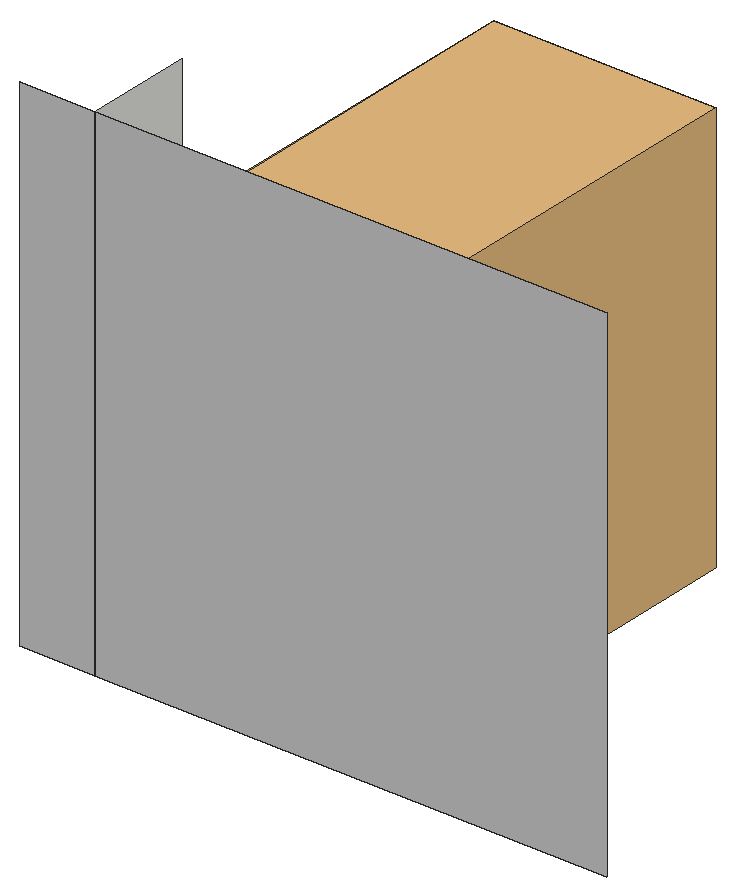
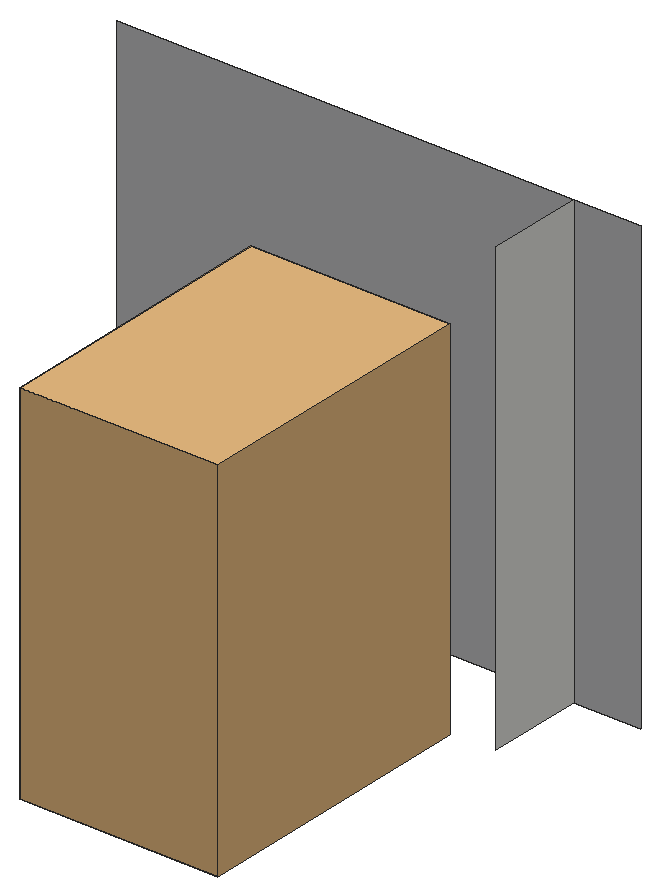
# SketchUp Ruby script. Lengths in inches.
U = 1.inch
M = Sketchup.active_model
def pt(a) = Geom::Point3d.new(a.map { |v| v * U })
def face(e, loops, mat)
  f = e.add_face(loops[0].map { |a| pt(a) })
  loops[1..].each { |l| e.add_face(l.map { |a| pt(a) }).erase! }
  f.material = f.back_material = mat if mat
  f
end
# faces: each face lists its corners as indices into pts; further lists are holes
def faces(e, pts, list, mat = nil) = list.each { |f| face(e, (f[0].is_a?(Array) ? f : [f]).map { |l| l.map { |i| pts[i] } }, mat) }
# xy, xz, yz: faces in a plane at the given z, y or x. An outline is a flat list of corners, or four numbers for a rectangle; further outlines are holes
def ring(l) = l.size == 4 ? [[l[0], l[1]], [l[2], l[1]], [l[2], l[3]], [l[0], l[3]]] : l.each_slice(2).to_a
def flat(e, list, mat, &to3) = list.each { |f| face(e, (f[0].is_a?(Array) ? f : [f]).map { |l| ring(l).map { |u, v| to3.(u, v) } }, mat) }
def xy(e, z, list, mat = nil) = flat(e, list, mat) { |x, y| [x, y, z] }
def xz(e, y, list, mat = nil) = flat(e, list, mat) { |x, z| [x, y, z] }
def yz(e, x, list, mat = nil) = flat(e, list, mat) { |y, z| [x, y, z] }
def lines(e, pts, list) = list.each { |a, b| e.add_line(pt(pts[a]), pt(pts[b])) }
# prism: a flat outline (further loops are holes) pulled along v
def prism(e, loops, v, mat = nil)
  f = face(e, loops, mat); d = Geom::Vector3d.new(v.map { |x| x * U })
  f.pushpull(f.normal.samedirection?(d) ? d.length : -d.length)
end
def box(e, o, s, mat = nil) = prism(e, [[o, [o[0] + s[0], o[1], o[2]], [o[0] + s[0], o[1] + s[1], o[2]], [o[0], o[1] + s[1], o[2]]]], [0, 0, s[2]], mat)
def at(x, y, z, deg = 0) = Geom::Transformation.translation(pt([x, y, z])) * Geom::Transformation.rotation(ORIGIN, Z_AXIS, deg.degrees)
def axes(o, x, y, z) = Geom::Transformation.new([*x, 0, *y, 0, *z, 0, *pt(o).to_a, 1])
def part(name) = M.definitions.add(name)
# library, detail: a bought-in or finely detailed component or shape, given as its bounding box
def library(name, o, s) = part(name).tap { |d| box(d.entities, o, s) }
def detail(e, o, s) = box(e.add_group.entities, o, s)
def put(e, d, t, mat = nil) = e.add_instance(d, t).tap { |i| i.material = mat if mat }
def group(e, t, mat = nil) = e.add_group.tap { |g| g.transformation = t; g.material = mat if mat }.entities
root = M.entities
M.materials.add("[Fencing Metal Straight]").color = [194, 195, 196]
c1 = library("chau cay",[-24.34,-109.24,0],[56.46,62.58,79.69])
xz(root,0,[[0,17.625,14.48,115.1875],[14.48,17.625,113.3,115.1875]],"[Fencing Metal Straight]")
yz(root,14.48,[[0,17.625,21.02,115.1875]])
put(root,c1,axes([42.5,130.99,17.625],[0.76,0,0],[0,1,0],[0,0,1]))
